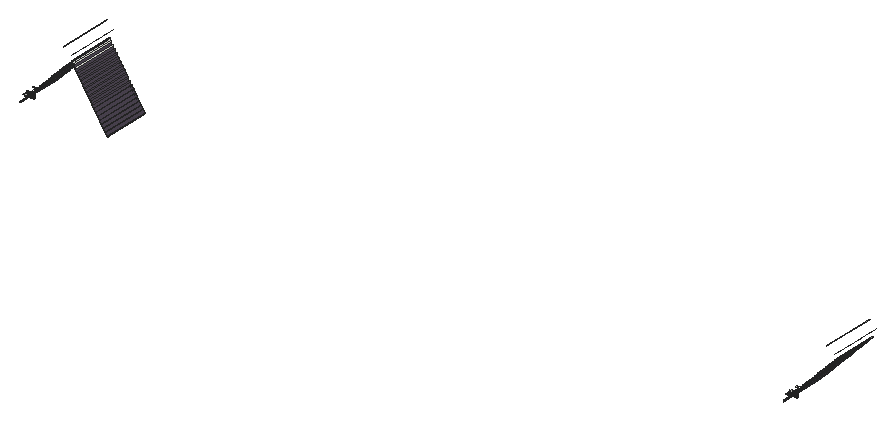
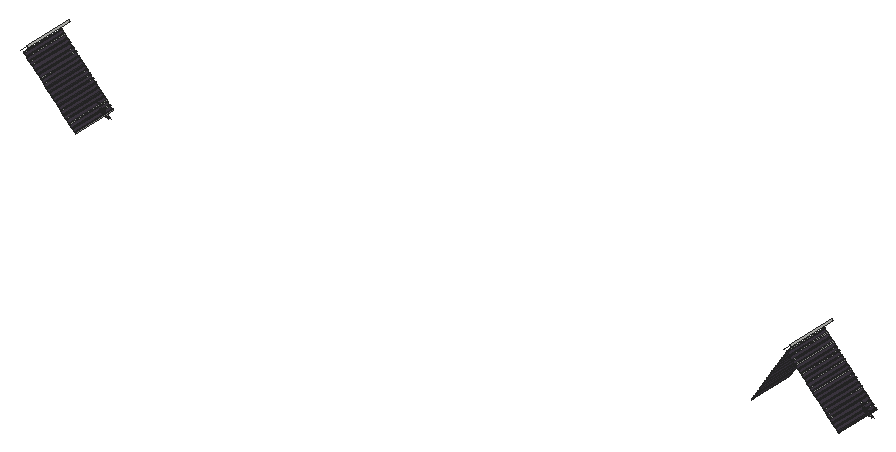
# SketchUp Ruby script. Lengths in inches.
U = 1.inch
M = Sketchup.active_model
def pt(a) = Geom::Point3d.new(a.map { |v| v * U })
def face(e, loops, mat)
  f = e.add_face(loops[0].map { |a| pt(a) })
  loops[1..].each { |l| e.add_face(l.map { |a| pt(a) }).erase! }
  f.material = f.back_material = mat if mat
  f
end
# faces: each face lists its corners as indices into pts; further lists are holes
def faces(e, pts, list, mat = nil) = list.each { |f| face(e, (f[0].is_a?(Array) ? f : [f]).map { |l| l.map { |i| pts[i] } }, mat) }
# xy, xz, yz: faces in a plane at the given z, y or x. An outline is a flat list of corners, or four numbers for a rectangle; further outlines are holes
def ring(l) = l.size == 4 ? [[l[0], l[1]], [l[2], l[1]], [l[2], l[3]], [l[0], l[3]]] : l.each_slice(2).to_a
def flat(e, list, mat, &to3) = list.each { |f| face(e, (f[0].is_a?(Array) ? f : [f]).map { |l| ring(l).map { |u, v| to3.(u, v) } }, mat) }
def xy(e, z, list, mat = nil) = flat(e, list, mat) { |x, y| [x, y, z] }
def xz(e, y, list, mat = nil) = flat(e, list, mat) { |x, z| [x, y, z] }
def yz(e, x, list, mat = nil) = flat(e, list, mat) { |y, z| [x, y, z] }
def lines(e, pts, list) = list.each { |a, b| e.add_line(pt(pts[a]), pt(pts[b])) }
# prism: a flat outline (further loops are holes) pulled along v
def prism(e, loops, v, mat = nil)
  f = face(e, loops, mat); d = Geom::Vector3d.new(v.map { |x| x * U })
  f.pushpull(f.normal.samedirection?(d) ? d.length : -d.length)
end
def box(e, o, s, mat = nil) = prism(e, [[o, [o[0] + s[0], o[1], o[2]], [o[0] + s[0], o[1] + s[1], o[2]], [o[0], o[1] + s[1], o[2]]]], [0, 0, s[2]], mat)
def at(x, y, z, deg = 0) = Geom::Transformation.translation(pt([x, y, z])) * Geom::Transformation.rotation(ORIGIN, Z_AXIS, deg.degrees)
def axes(o, x, y, z) = Geom::Transformation.new([*x, 0, *y, 0, *z, 0, *pt(o).to_a, 1])
def part(name) = M.definitions.add(name)
# library, detail: a bought-in or finely detailed component or shape, given as its bounding box
def library(name, o, s) = part(name).tap { |d| box(d.entities, o, s) }
def detail(e, o, s) = box(e.add_group.entities, o, s)
def put(e, d, t, mat = nil) = e.add_instance(d, t).tap { |i| i.material = mat if mat }
def group(e, t, mat = nil) = e.add_group.tap { |g| g.transformation = t; g.material = mat if mat }.entities
root = M.entities
M.materials.add("[Color M06]").color = [79, 71, 84]
xy(root,386.399,[[494.351,480.141,496.663,480.766],[497.263,480.141,499.575,480.766],[1380.815,480.141,1383.127,480.766],[1383.727,480.141,1386.039,480.766]])
xy(root,386.837,[[494.535,480.141,496.663,480.766],[497.263,480.141,499.575,480.766],[1380.999,480.141,1383.127,480.766],[1383.727,480.141,1386.039,480.766]])
xy(root,389.149,[[497.263,480.141,499.575,480.766],[1383.727,480.141,1386.039,480.766]])
xy(root,389.587,[[497.263,480.141,499.575,480.766],[1383.727,480.141,1386.039,480.766]])
xy(root,391.899,[[499.28,480.141,499.575,480.766],[1385.744,480.141,1386.039,480.766]])
xy(root,397.749,[[498.037,480.141,500.287,480.766],[1384.501,480.141,1386.751,480.766]])
xz(root,467.1875,[[554.756,447.754,555.124,447.99,553.555,450.4375,553.246,450.109],[553.246,450.109,553.555,450.4375,553.187,450.201],[1439.71,450.109,1440.019,450.4375,1439.651,450.201]])
xz(root,480.141,[[488.527,385.926,488.97,386.399,488.527,386.399],[1374.991,385.926,1375.434,386.399,1374.991,386.399],[491.439,386.283,491.548,386.399,491.439,386.399],[1377.903,386.283,1378.012,386.399,1377.903,386.399],[487.765,386.837,487.927,386.837,487.927,387.008],
  [488.527,386.837,490.359,386.837,490.839,387.346,490.839,389.149,489.942,389.149,488.527,387.645],[490.359,386.837,490.839,386.837,490.839,387.346],[491.439,386.837,493.751,386.837,493.751,389.149,492.536,389.149,491.439,387.983],[494.351,386.837,494.535,386.837,496.663,389.107,496.663,389.149,494.351,389.149],[1374.229,386.837,1374.391,386.837,1374.391,387.008],
  [1374.991,386.837,1376.823,386.837,1377.303,387.346,1377.303,389.149,1376.406,389.149,1374.991,387.645],[1376.823,386.837,1377.303,386.837,1377.303,387.346],[1377.903,386.837,1380.215,386.837,1380.215,389.149,1379,389.149,1377.903,387.983],[1380.815,386.837,1380.999,386.837,1383.127,389.107,1383.127,389.149,1380.815,389.149],[491.439,389.033,491.548,389.149,491.439,389.149],
  [1377.903,389.033,1378.012,389.149,1377.903,389.149],[490.354,389.587,490.839,389.587,490.839,390.102],[491.439,389.587,492.948,389.587,493.751,390.44,493.751,391.899,492.531,391.899,491.439,390.739],[492.948,389.587,493.751,389.587,493.751,390.44],[494.351,389.587,494.535,389.587,496.663,391.857,496.663,391.899,495.125,391.899,494.351,391.077],
  [494.535,389.587,496.663,389.587,496.663,391.857],[1376.818,389.587,1377.303,389.587,1377.303,390.102],[1377.903,389.587,1379.412,389.587,1380.215,390.44,1380.215,391.899,1378.995,391.899,1377.903,390.739],[1379.412,389.587,1380.215,389.587,1380.215,390.44],[1380.815,389.587,1380.999,389.587,1383.127,391.857,1383.127,391.899,1381.589,391.899,1380.815,391.077],
  [1380.999,389.587,1383.127,389.587,1383.127,391.857],[497.263,389.747,499.28,391.899,497.263,391.899],[1383.727,389.747,1385.744,391.899,1383.727,391.899],[494.351,391.077,495.125,391.899,494.351,391.899],[1380.815,391.077,1381.589,391.899,1380.815,391.899]])
xz(root,519.6875,[[594.777,385.328,594.721,385.417,595.089,385.653,595.146,385.565],[592.585,388.748,592.528,388.837,592.896,389.073,592.953,388.985],[590.392,392.168,590.336,392.257,590.704,392.493,590.761,392.405],[588.2,395.588,588.143,395.677,588.511,395.913,588.568,395.825],[586.007,399.009,585.95,399.097,586.319,399.333,586.375,399.245],
  [583.815,402.429,583.758,402.517,584.126,402.753,584.183,402.665],[581.622,405.849,581.565,405.937,581.933,406.173,581.99,406.085],[579.429,409.269,579.373,409.357,579.741,409.593,579.798,409.505],[577.237,412.689,577.18,412.777,577.548,413.013,577.605,412.925],[575.044,416.109,574.987,416.197,575.356,416.433,575.412,416.345],
  [572.852,419.529,572.795,419.617,573.163,419.853,573.22,419.765],[570.659,422.949,570.602,423.037,570.97,423.273,571.027,423.185],[568.466,426.369,568.41,426.457,568.778,426.693,568.835,426.605],[566.274,429.789,566.217,429.877,566.585,430.113,566.642,430.025],[564.081,433.209,564.024,433.297,564.393,433.533,564.449,433.445],
  [561.889,436.629,561.832,436.717,562.2,436.953,562.257,436.865],[559.696,440.049,559.639,440.137,560.008,440.373,560.064,440.285],[557.503,443.469,557.447,443.557,557.815,443.793,557.872,443.705],[555.311,446.889,555.254,446.977,555.622,447.213,555.679,447.125]])
yz(root,496.663,[[480.141,386.837,480.766,389.107]])
yz(root,497.263,[[480.141,386.837,480.766,389.149],[480.141,389.587,480.766,389.747]])
yz(root,499.575,[[480.141,386.837,480.766,389.149],[480.141,389.587,480.766,391.899]])
yz(root,1383.127,[[480.141,386.837,480.766,389.107]])
yz(root,1383.727,[[480.141,386.837,480.766,389.149],[480.141,389.587,480.766,389.747]])
yz(root,1386.039,[[480.141,386.837,480.766,389.149],[480.141,389.587,480.766,391.899]])
p = [[595.146,519.6875,385.565],[595.146,521.5625,385.565],[594.777,521.5625,385.328],[594.777,519.6875,385.328],[595.089,467.1875,385.653],[595.089,519.6875,385.653],
  [594.721,519.6875,385.417],[594.721,467.1875,385.417],[592.528,467.1875,388.837],[592.528,519.6875,388.837],[592.585,519.6875,388.748],[592.585,521.5625,388.748],
  [594.223,521.5625,386.194],[594.223,467.1875,386.194],[594.591,521.5625,386.43],[594.591,467.1875,386.43],[493.603,521.5625,386.746],[493.603,467.1875,386.746],
  [494.058,467.1875,386.318],[494.058,521.5625,386.318],[1380.067,521.5625,386.746],[1380.067,467.1875,386.746],[1380.522,467.1875,386.318],[1380.522,521.5625,386.318],
  [494.48,521.5625,387.679],[494.48,467.1875,387.679],[1380.944,521.5625,387.679],[1380.944,467.1875,387.679],[496.663,480.141,389.107],[494.535,480.141,386.837],
  [494.535,480.766,386.837],[496.663,480.766,389.107],[1383.127,480.141,389.107],[1380.999,480.141,386.837],[1380.999,480.766,386.837],[1383.127,480.766,389.107],
  [494.935,521.5625,387.25],[494.935,467.1875,387.25],[497.357,521.5625,389.822],[497.357,467.1875,389.822],[1381.399,521.5625,387.25],[1381.399,467.1875,387.25],
  [1383.821,521.5625,389.822],[1383.821,467.1875,389.822],[592.953,519.6875,388.985],[592.953,521.5625,388.985],[592.896,467.1875,389.073],[592.896,519.6875,389.073],
  [590.336,467.1875,392.257],[590.336,519.6875,392.257],[590.392,519.6875,392.168],[590.392,521.5625,392.168],[592.03,521.5625,389.614],[592.03,467.1875,389.614],
  [592.398,521.5625,389.85],[592.398,467.1875,389.85],[499.28,480.141,391.899],[497.263,480.141,389.747],[497.263,480.766,389.747],[499.28,480.766,391.899],
  [1385.744,480.141,391.899],[1383.727,480.141,389.747],[1383.727,480.766,389.747],[1385.744,480.766,391.899],[496.901,521.5625,390.251],[496.901,467.1875,390.251],
  [1383.365,521.5625,390.251],[1383.365,467.1875,390.251],[497.779,521.5625,391.183],[497.779,467.1875,391.183],[1384.243,521.5625,391.183],[1384.243,467.1875,391.183],
  [498.234,521.5625,390.754],[498.234,467.1875,390.754],[500.655,521.5625,393.327],[500.655,467.1875,393.327],[1384.698,521.5625,390.754],[1384.698,467.1875,390.754],
  [1387.119,521.5625,393.327],[1387.119,467.1875,393.327],[590.704,467.1875,392.493],[590.704,519.6875,392.493],[588.143,467.1875,395.677],[588.143,519.6875,395.677],
  [588.2,519.6875,395.588],[588.2,521.5625,395.588],[589.837,521.5625,393.034],[589.837,467.1875,393.034],[590.206,521.5625,393.27],[590.206,467.1875,393.27],
  [500.2,521.5625,393.755],[500.2,467.1875,393.755],[1386.664,521.5625,393.755],[1386.664,467.1875,393.755],[501.077,521.5625,394.687],[501.077,467.1875,394.687],
  [1387.541,521.5625,394.687],[1387.541,467.1875,394.687],[501.533,521.5625,394.259],[501.533,467.1875,394.259],[503.954,521.5625,396.831],[503.954,467.1875,396.831],
  [1387.997,521.5625,394.259],[1387.997,467.1875,394.259],[1390.418,521.5625,396.831],[1390.418,467.1875,396.831],[588.511,467.1875,395.913],[588.511,519.6875,395.913],
  [585.95,467.1875,399.097],[585.95,519.6875,399.097],[586.007,519.6875,399.009],[586.007,521.5625,399.009],[587.645,521.5625,396.454],[587.645,467.1875,396.454],
  [588.013,521.5625,396.69],[588.013,467.1875,396.69],[503.499,521.5625,397.259],[503.499,467.1875,397.259],[1389.963,521.5625,397.259],[1389.963,467.1875,397.259],
  [504.376,521.5625,398.191],[504.376,467.1875,398.191],[1390.84,521.5625,398.191],[1390.84,467.1875,398.191],[504.831,521.5625,397.763],[504.831,467.1875,397.763],
  [507.252,521.5625,400.335],[507.252,467.1875,400.335],[1391.295,521.5625,397.763],[1391.295,467.1875,397.763],[1393.716,521.5625,400.335],[1393.716,467.1875,400.335],
  [586.319,467.1875,399.333],[586.319,519.6875,399.333],[583.758,467.1875,402.517],[583.758,519.6875,402.517],[583.815,519.6875,402.429],[583.815,521.5625,402.429],
  [585.452,521.5625,399.874],[585.452,467.1875,399.874],[585.821,521.5625,400.11],[585.821,467.1875,400.11],[506.797,521.5625,400.763],[506.797,467.1875,400.763],
  [1393.261,521.5625,400.763],[1393.261,467.1875,400.763],[507.675,521.5625,401.696],[507.675,467.1875,401.696],[1394.139,521.5625,401.696],[1394.139,467.1875,401.696],
  [508.13,521.5625,401.267],[508.13,467.1875,401.267],[510.551,521.5625,403.839],[510.551,467.1875,403.839],[1394.594,521.5625,401.267],[1394.594,467.1875,401.267],
  [1397.015,521.5625,403.839],[1397.015,467.1875,403.839],[584.126,467.1875,402.753],[584.126,519.6875,402.753],[581.565,467.1875,405.937],[581.565,519.6875,405.937],
  [581.622,519.6875,405.849],[581.622,521.5625,405.849],[583.26,521.5625,403.294],[583.26,467.1875,403.294],[583.628,521.5625,403.53],[583.628,467.1875,403.53],
  [510.096,521.5625,404.268],[510.096,467.1875,404.268],[1396.56,521.5625,404.268],[1396.56,467.1875,404.268],[510.973,521.5625,405.2],[510.973,467.1875,405.2],
  [1397.437,521.5625,405.2],[1397.437,467.1875,405.2],[511.428,521.5625,404.771],[511.428,467.1875,404.771],[513.849,521.5625,407.344],[513.849,467.1875,407.344],
  [1397.892,521.5625,404.771],[1397.892,467.1875,404.771],[1400.313,521.5625,407.344],[1400.313,467.1875,407.344],[581.933,467.1875,406.173],[581.933,519.6875,406.173],
  [579.373,467.1875,409.357],[579.373,519.6875,409.357],[579.429,519.6875,409.269],[579.429,521.5625,409.269],[581.067,521.5625,406.714],[581.067,467.1875,406.714],
  [581.435,521.5625,406.95],[581.435,467.1875,406.95],[513.394,521.5625,407.772],[513.394,467.1875,407.772],[1399.858,521.5625,407.772],[1399.858,467.1875,407.772],
  [514.272,521.5625,408.704],[514.272,467.1875,408.704],[1400.736,521.5625,408.704],[1400.736,467.1875,408.704],[514.727,521.5625,408.276],[514.727,467.1875,408.276],
  [517.148,521.5625,410.848],[517.148,467.1875,410.848],[1401.191,521.5625,408.276],[1401.191,467.1875,408.276],[1403.612,521.5625,410.848],[1403.612,467.1875,410.848],
  [579.741,467.1875,409.593],[579.741,519.6875,409.593],[577.18,467.1875,412.777],[577.18,519.6875,412.777],[577.237,519.6875,412.689],[577.237,521.5625,412.689],
  [577.535,521.5625,412.223],[577.687,521.5625,411.987],[578.874,521.5625,410.134],[578.874,467.1875,410.134],[579.243,521.5625,410.37],[579.243,467.1875,410.37],
  [516.693,521.5625,411.276],[516.693,467.1875,411.276],[1403.157,521.5625,411.276],[1403.157,467.1875,411.276],[517.57,521.5625,412.208],[517.57,467.1875,412.208],
  [1404.034,521.5625,412.208],[1404.034,467.1875,412.208],[518.025,521.5625,411.78],[518.025,467.1875,411.78],[520.446,521.5625,414.352],[520.446,467.1875,414.352],
  [1404.489,521.5625,411.78],[1404.489,467.1875,411.78],[1406.91,521.5625,414.352],[1406.91,467.1875,414.352],[577.605,519.6875,412.925],[577.605,521.5625,412.925],
  [577.548,467.1875,413.013],[577.548,519.6875,413.013],[577.05,467.1875,413.79],[577.05,521.5625,413.79],[574.987,467.1875,416.197],[574.987,519.6875,416.197],
  [575.044,519.6875,416.109],[575.044,521.5625,416.109],[575.494,521.5625,415.407],[576.682,521.5625,413.554],[576.682,467.1875,413.554],[519.991,521.5625,414.78],
  [519.991,467.1875,414.78],[1406.455,521.5625,414.78],[1406.455,467.1875,414.78],[520.869,521.5625,415.713],[520.869,467.1875,415.713],[1407.333,521.5625,415.713],
  [1407.333,467.1875,415.713],[521.324,521.5625,415.284],[521.324,467.1875,415.284],[523.745,521.5625,417.856],[523.745,467.1875,417.856],[1407.788,521.5625,415.284],
  [1407.788,467.1875,415.284],[1410.209,521.5625,417.856],[1410.209,467.1875,417.856],[575.412,519.6875,416.345],[575.412,521.5625,416.345],[575.356,467.1875,416.433],
  [575.356,519.6875,416.433],[574.858,467.1875,417.21],[574.858,521.5625,417.21],[572.795,467.1875,419.617],[572.795,519.6875,419.617],[572.852,519.6875,419.529],
  [572.852,521.5625,419.529],[573.301,521.5625,418.827],[574.489,521.5625,416.974],[574.489,467.1875,416.974],[523.29,521.5625,418.285],[523.29,467.1875,418.285],
  [1409.754,521.5625,418.285],[1409.754,467.1875,418.285],[524.167,521.5625,419.217],[524.167,467.1875,419.217],[1410.631,521.5625,419.217],[1410.631,467.1875,419.217],
  [524.622,521.5625,418.788],[524.622,467.1875,418.788],[527.043,521.5625,421.361],[527.043,467.1875,421.361],[1411.086,521.5625,418.788],[1411.086,467.1875,418.788],
  [1413.507,521.5625,421.361],[1413.507,467.1875,421.361],[573.22,519.6875,419.765],[573.22,521.5625,419.765],[573.163,467.1875,419.853],[573.163,519.6875,419.853],
  [572.665,467.1875,420.63],[572.665,521.5625,420.63],[570.602,467.1875,423.037],[570.602,519.6875,423.037],[570.659,519.6875,422.949],[570.659,521.5625,422.949],
  [571.109,521.5625,422.247],[572.297,521.5625,420.394],[572.297,467.1875,420.394],[526.588,521.5625,421.789],[526.588,467.1875,421.789],[1413.052,521.5625,421.789],
  [1413.052,467.1875,421.789],[527.466,521.5625,422.721],[527.466,467.1875,422.721],[1413.93,521.5625,422.721],[1413.93,467.1875,422.721],[527.921,521.5625,422.293],
  [527.921,467.1875,422.293],[530.342,521.5625,424.865],[530.342,467.1875,424.865],[1414.385,521.5625,422.293],[1414.385,467.1875,422.293],[1416.806,521.5625,424.865],
  [1416.806,467.1875,424.865],[571.027,519.6875,423.185],[571.027,521.5625,423.185],[570.97,467.1875,423.273],[570.97,519.6875,423.273],[570.472,467.1875,424.05],
  [570.472,521.5625,424.05],[568.41,467.1875,426.457],[568.41,519.6875,426.457],[568.466,519.6875,426.369],[568.466,521.5625,426.369],[568.916,521.5625,425.667],
  [570.104,521.5625,423.814],[570.104,467.1875,423.814],[529.887,521.5625,425.293],[529.887,467.1875,425.293],[1416.351,521.5625,425.293],[1416.351,467.1875,425.293],
  [530.764,521.5625,426.225],[530.764,467.1875,426.225],[1417.228,521.5625,426.225],[1417.228,467.1875,426.225],[531.219,521.5625,425.797],[531.219,467.1875,425.797],
  [533.641,521.5625,428.369],[533.641,467.1875,428.369],[1417.683,521.5625,425.797],[1417.683,467.1875,425.797],[1420.105,521.5625,428.369],[1420.105,467.1875,428.369],
  [568.835,519.6875,426.605],[568.835,521.5625,426.605],[568.778,467.1875,426.693],[568.778,519.6875,426.693],[568.28,467.1875,427.47],[568.28,521.5625,427.47],
  [566.217,467.1875,429.877],[566.217,519.6875,429.877],[566.274,519.6875,429.789],[566.274,521.5625,429.789],[566.724,521.5625,429.087],[567.911,521.5625,427.234],
  [567.911,467.1875,427.234],[533.185,521.5625,428.797],[533.185,467.1875,428.797],[1419.649,521.5625,428.797],[1419.649,467.1875,428.797],[534.063,521.5625,429.73],
  [534.063,467.1875,429.73],[1420.527,521.5625,429.73],[1420.527,467.1875,429.73],[534.518,521.5625,429.301],[534.518,467.1875,429.301],[536.939,521.5625,431.873],
  [536.939,467.1875,431.873],[1420.982,521.5625,429.301],[1420.982,467.1875,429.301],[1423.403,521.5625,431.873],[1423.403,467.1875,431.873],[566.642,519.6875,430.025],
  [566.642,521.5625,430.025],[566.585,467.1875,430.113],[566.585,519.6875,430.113],[566.087,467.1875,430.89],[566.087,521.5625,430.89],[564.024,467.1875,433.297],
  [564.024,519.6875,433.297],[564.081,519.6875,433.209],[564.081,521.5625,433.209],[564.531,521.5625,432.507],[565.719,521.5625,430.654],[565.719,467.1875,430.654],
  [536.484,521.5625,432.302],[536.484,467.1875,432.302],[1422.948,521.5625,432.302],[1422.948,467.1875,432.302],[537.361,521.5625,433.234],[537.361,467.1875,433.234],
  [1423.825,521.5625,433.234],[1423.825,467.1875,433.234],[537.817,521.5625,432.805],[537.817,467.1875,432.805],[540.238,521.5625,435.378],[540.238,467.1875,435.378],
  [1424.281,521.5625,432.805],[1424.281,467.1875,432.805],[1426.702,521.5625,435.378],[1426.702,467.1875,435.378],[564.449,519.6875,433.445],[564.449,521.5625,433.445],
  [564.393,467.1875,433.533],[564.393,519.6875,433.533],[563.895,467.1875,434.31],[563.895,521.5625,434.31],[561.832,467.1875,436.717],[561.832,519.6875,436.717],
  [561.889,519.6875,436.629],[561.889,521.5625,436.629],[562.338,521.5625,435.927],[563.526,521.5625,434.074],[563.526,467.1875,434.074],[539.783,521.5625,435.806],
  [539.783,467.1875,435.806],[1426.247,521.5625,435.806],[1426.247,467.1875,435.806],[540.66,521.5625,436.738],[540.66,467.1875,436.738],[1427.124,521.5625,436.738],
  [1427.124,467.1875,436.738],[541.115,521.5625,436.31],[541.115,467.1875,436.31],[543.536,521.5625,438.882],[543.536,467.1875,438.882],[1427.579,521.5625,436.31],
  [1427.579,467.1875,436.31],[1430,521.5625,438.882],[1430,467.1875,438.882],[562.257,519.6875,436.865],[562.257,521.5625,436.865],[562.2,467.1875,436.953],
  [562.2,519.6875,436.953],[561.702,467.1875,437.73],[561.702,521.5625,437.73],[559.639,467.1875,440.137],[559.639,519.6875,440.137],[559.696,519.6875,440.049],
  [559.696,521.5625,440.049],[560.146,521.5625,439.347],[561.334,521.5625,437.494],[561.334,467.1875,437.494],[543.081,521.5625,439.31],[543.081,467.1875,439.31],
  [1429.545,521.5625,439.31],[1429.545,467.1875,439.31],[543.959,521.5625,440.242],[543.959,467.1875,440.242],[1430.423,521.5625,440.242],[1430.423,467.1875,440.242],
  [544.414,521.5625,439.814],[544.414,467.1875,439.814],[546.835,521.5625,442.386],[546.835,467.1875,442.386],[1430.878,521.5625,439.814],[1430.878,467.1875,439.814],
  [1433.299,521.5625,442.386],[1433.299,467.1875,442.386],[560.064,519.6875,440.285],[560.064,521.5625,440.285],[560.008,467.1875,440.373],[560.008,519.6875,440.373],
  [559.509,467.1875,441.15],[559.509,521.5625,441.15],[557.447,467.1875,443.557],[557.447,519.6875,443.557],[557.503,519.6875,443.469],[557.503,521.5625,443.469],
  [557.953,521.5625,442.767],[559.141,521.5625,440.914],[559.141,467.1875,440.914],[546.38,521.5625,442.814],[546.38,467.1875,442.814],[1432.844,521.5625,442.814],
  [1432.844,467.1875,442.814],[547.257,521.5625,443.747],[547.257,467.1875,443.747],[1433.721,521.5625,443.747],[1433.721,467.1875,443.747],[547.712,521.5625,443.318],
  [547.712,467.1875,443.318],[550.133,521.5625,445.89],[550.133,467.1875,445.89],[1434.176,521.5625,443.318],[1434.176,467.1875,443.318],[1436.597,521.5625,445.89],
  [1436.597,467.1875,445.89],[557.872,519.6875,443.705],[557.872,521.5625,443.705],[557.815,467.1875,443.793],[557.815,519.6875,443.793],[557.317,467.1875,444.57],
  [557.317,521.5625,444.57],[555.254,467.1875,446.977],[555.254,519.6875,446.977],[555.311,519.6875,446.889],[555.311,521.5625,446.889],[555.761,521.5625,446.187],
  [556.948,521.5625,444.334],[556.948,467.1875,444.334],[549.678,521.5625,446.319],[549.678,467.1875,446.319],[1436.142,521.5625,446.319],[1436.142,467.1875,446.319],
  [550.556,521.5625,447.251],[550.556,467.1875,447.251],[1437.02,521.5625,447.251],[1437.02,467.1875,447.251],[551.011,521.5625,446.822],[551.011,467.1875,446.822],
  [553.432,521.5625,449.395],[553.432,467.1875,449.395],[1437.475,521.5625,446.822],[1437.475,467.1875,446.822],[1439.896,521.5625,449.395],[1439.896,467.1875,449.395],
  [555.679,519.6875,447.125],[555.679,521.5625,447.125],[555.622,467.1875,447.213],[555.622,519.6875,447.213],[555.124,467.1875,447.99],[555.124,521.5625,447.99],
  [553.568,521.5625,449.607],[554.756,521.5625,447.754],[554.756,467.1875,447.754],[553.246,467.1875,450.109],[553.187,467.1875,450.201],[553.187,521.5625,450.201],
  [553.246,521.5625,450.109],[553.936,521.5625,449.843],[553.555,521.5625,450.4375],[553.555,467.1875,450.4375],[552.977,521.5625,449.823],[552.977,467.1875,449.823],
  [1439.441,521.5625,449.823],[1439.441,467.1875,449.823],[1439.71,467.1875,450.109],[1439.71,521.5625,450.109],[1440.019,521.5625,450.4375],[1440.019,467.1875,450.4375],
  [1439.651,521.5625,450.201],[1439.651,467.1875,450.201],[553.486,521.5625,450.545],[553.43,467.1875,450.633],[553.43,519.6875,450.633],[553.486,519.6875,450.545],
  [1439.95,521.5625,450.545],[1439.894,467.1875,450.633],[1439.894,519.6875,450.633],[1439.95,519.6875,450.545],[543.649,528.483,461.307],[543.649,467.1875,461.307],
  [544.977,467.1875,462.718],[544.977,528.483,462.718],[1430.113,528.483,461.307],[1430.113,467.1875,461.307],[1431.441,467.1875,462.718],[1431.441,528.483,462.718],
  [1386.175,480.141,395.86],[1385.317,480.141,395.86],[1381.589,480.141,391.899],[1374.991,480.141,384.89],[1374.991,480.141,385.926],[1378.012,480.141,389.149],
  [1379,480.141,389.149],[1375.434,480.141,386.399],[1376.412,480.141,386.399],[1374.391,480.141,388.036],[1374.391,480.141,387.008],[1375.434,480.141,389.149],
  [1376.406,480.141,389.149],[1374.991,480.141,387.645],[1374.991,480.141,388.676],[1374.229,480.141,386.837],[1373.267,480.141,386.837],[1376.823,480.141,386.837],
  [1377.903,480.141,387.983],[1377.303,480.141,387.346],[1377.903,480.141,389.033],[1376.406,480.141,391.899],[1376.412,480.141,391.899],[1380.815,480.141,391.077],
  [1380.215,480.141,390.44],[1379.412,480.141,389.587],[1376.818,480.141,389.587],[1375.844,480.141,389.587],[1372.857,480.141,386.399],[1373.818,480.141,386.399],
  [1372.079,480.141,385.569],[1438.978,528.483,455.623],[1438.978,467.1875,455.623],[499.711,480.141,395.86],[498.853,480.141,395.86],[495.125,480.141,391.899],
  [552.514,528.483,455.623],[552.514,467.1875,455.623],[486.393,480.141,386.399],[487.354,480.141,386.399],[491.548,480.141,389.149],[492.536,480.141,389.149],
  [488.97,480.141,386.399],[489.948,480.141,386.399],[485.615,480.141,385.569],[490.354,480.141,389.587],[489.38,480.141,389.587],[494.351,480.141,391.077],
  [493.751,480.141,390.44],[492.948,480.141,389.587],[488.527,480.141,387.645],[488.527,480.141,388.676],[487.765,480.141,386.837],[486.803,480.141,386.837],
  [488.97,480.141,389.149],[489.942,480.141,389.149],[491.439,480.141,387.983],[491.439,480.141,389.033],[490.359,480.141,386.837],[490.839,480.141,387.346],
  [487.927,480.141,388.036],[487.927,480.141,387.008],[489.942,480.141,391.899],[489.948,480.141,391.899],[488.527,480.141,384.89],[488.527,480.141,385.926]]
faces(root,p,[[0,1,2,3],[4,5,6,7],[14,15,13,12],[16,17,18,19],[20,21,22,23],[28,29,30,31],[32,33,34,35],[44,45,11,10],
  [46,47,9,8],[54,55,53,52],[56,57,58,59],[60,61,62,63],[64,65,39,38],[66,67,43,42],[69,68,72,73],[71,70,76,77],
  [80,81,49,48],[88,89,87,86],[90,91,75,74],[92,93,79,78],[95,94,98,99],[97,96,102,103],[106,107,83,82],[114,115,113,112],
  [116,117,101,100],[118,119,105,104],[121,120,124,125],[123,122,128,129],[132,133,109,108],[140,141,139,138],[142,143,127,126],[144,145,131,130],
  [158,159,135,134],[166,167,165,164],[168,169,153,152],[170,171,157,156],[184,185,161,160],[192,193,191,190],[194,195,179,178],[196,197,183,182],
  [210,211,187,186],[220,221,219,218],[222,223,205,204],[224,225,209,208],[238,239,215,214],[240,241,213,212],[243,242,250,249],[251,252,233,232],
  [253,254,237,236],[267,268,247,246],[269,270,245,244],[272,271,279,278],[280,281,262,261],[282,283,266,265],[296,297,276,275],[298,299,274,273],
  [301,300,308,307],[309,310,291,290],[311,312,295,294],[325,326,305,304],[327,328,303,302],[330,329,337,336],[338,339,320,319],[340,341,324,323],
  [354,355,334,333],[356,357,332,331],[359,358,366,365],[367,368,349,348],[369,370,353,352],[372,371,375,376],[374,373,379,380],[383,384,363,362],
  [385,386,361,360],[388,387,395,394],[396,397,378,377],[398,399,382,381],[401,400,404,405],[403,402,408,409],[412,413,392,391],[414,415,390,389],
  [417,416,424,423],[425,426,407,406],[427,428,411,410],[430,429,433,434],[432,431,437,438],[441,442,421,420],[443,444,419,418],[446,445,453,452],
  [454,455,436,435],[456,457,440,439],[459,458,462,463],[461,460,466,467],[470,471,450,449],[472,473,448,447],[483,484,465,464],[485,486,469,468],
  [488,487,491,492],[490,489,495,496],[499,500,479,478],[501,502,477,476],[501,503,504,500,499,502],[512,513,494,493],[514,515,498,497],[517,516,520,521],
  [519,518,524,525],[528,529,508,507],[530,531,506,505],[530,532,533,529,528,531],[533,541,542,543,532],[544,545,523,522],[546,547,527,526],[537,545,544,540,542,543],
  [548,547,546,549,550,551],[543,542,539,538],[551,550,552,553],[554,542,543,555,556,557],[558,550,551,559,560,561],[562,563,564,565],[566,567,568,569]])
faces(root,p,[[8,9,10,11,12,13],[16,24,25,17],[20,26,27,21],[25,24,36,37],[36,38,39,37],[27,26,40,41],[40,42,43,41],[48,49,50,51,52,53],
  [64,68,69,65],[66,70,71,67],[72,74,75,73],[76,78,79,77],[82,83,84,85,86,87],[90,94,95,91],[92,96,97,93],[98,100,101,99],
  [102,104,105,103],[108,109,110,111,112,113],[116,120,121,117],[118,122,123,119],[124,126,127,125],[128,130,131,129],[134,135,136,137,138,139],[142,146,147,143],
  [144,148,149,145],[147,146,150,151],[150,152,153,151],[149,148,154,155],[154,156,157,155],[160,161,162,163,164,165],[168,172,173,169],[170,174,175,171],
  [173,172,176,177],[176,178,179,177],[175,174,180,181],[180,182,183,181],[186,187,188,189,190,191],[194,198,199,195],[196,200,201,197],[199,198,202,203],
  [202,204,205,203],[201,200,206,207],[206,208,209,207],[212,213,214,215,216,217,218,219],[222,226,227,223],[224,228,229,225],[227,226,230,231],[230,232,233,231],
  [229,228,234,235],[234,236,237,235],[240,242,243,239,238,241],[244,245,246,247,248,249,250],[251,255,256,252],[253,257,258,254],[256,255,259,260],[259,261,262,260],
  [258,257,263,264],[263,265,266,264],[269,271,272,268,267,270],[273,274,275,276,277,278,279],[280,284,285,281],[282,286,287,283],[285,284,288,289],[288,290,291,289],
  [287,286,292,293],[292,294,295,293],[298,300,301,297,296,299],[302,303,304,305,306,307,308],[309,313,314,310],[311,315,316,312],[314,313,317,318],[317,319,320,318],
  [316,315,321,322],[321,323,324,322],[327,329,330,326,325,328],[331,332,333,334,335,336,337],[338,342,343,339],[340,344,345,341],[343,342,346,347],[346,348,349,347],
  [345,344,350,351],[350,352,353,351],[356,358,359,355,354,357],[360,361,362,363,364,365,366],[367,371,372,368],[369,373,374,370],[375,377,378,376],[379,381,382,380],
  [385,387,388,384,383,386],[389,390,391,392,393,394,395],[396,400,401,397],[398,402,403,399],[404,406,407,405],[408,410,411,409],[414,416,417,413,412,415],[418,419,420,421,422,423,424],
  [425,429,430,426],[427,431,432,428],[433,435,436,434],[437,439,440,438],[443,445,446,442,441,444],[447,448,449,450,451,452,453],[454,458,459,455],[456,460,461,457],
  [462,464,465,463],[466,468,469,467],[472,474,475,471,470,473],[476,477,478,479,480,481,482],[475,474,482,481],[483,487,488,484],[485,489,490,486],[491,493,494,492],
  [495,497,498,496],[505,506,507,508,509,510,511],[504,503,511,510],[512,516,517,513],[514,518,519,515],[520,522,523,521],[524,526,527,525],[534,535,536,537,538,539,540],
  [533,532,536,535]],"[Color M06]")
lines(root,p,[[570,571],[571,572],[573,574],[575,576],[577,578],[579,580],[581,582],[583,584],[585,586],[587,578],[588,589],[588,590],
  [591,592],[593,594],[595,576],[596,597],[598,599],[598,600],[601,602],[603,604],[604,605],[606,607],[608,609],[610,611],
  [612,613],[608,614],[615,616],[617,618],[619,611],[620,621],[622,623],[624,625],[626,627],[628,613],[626,629],[630,631],
  [632,633],[634,635]])
